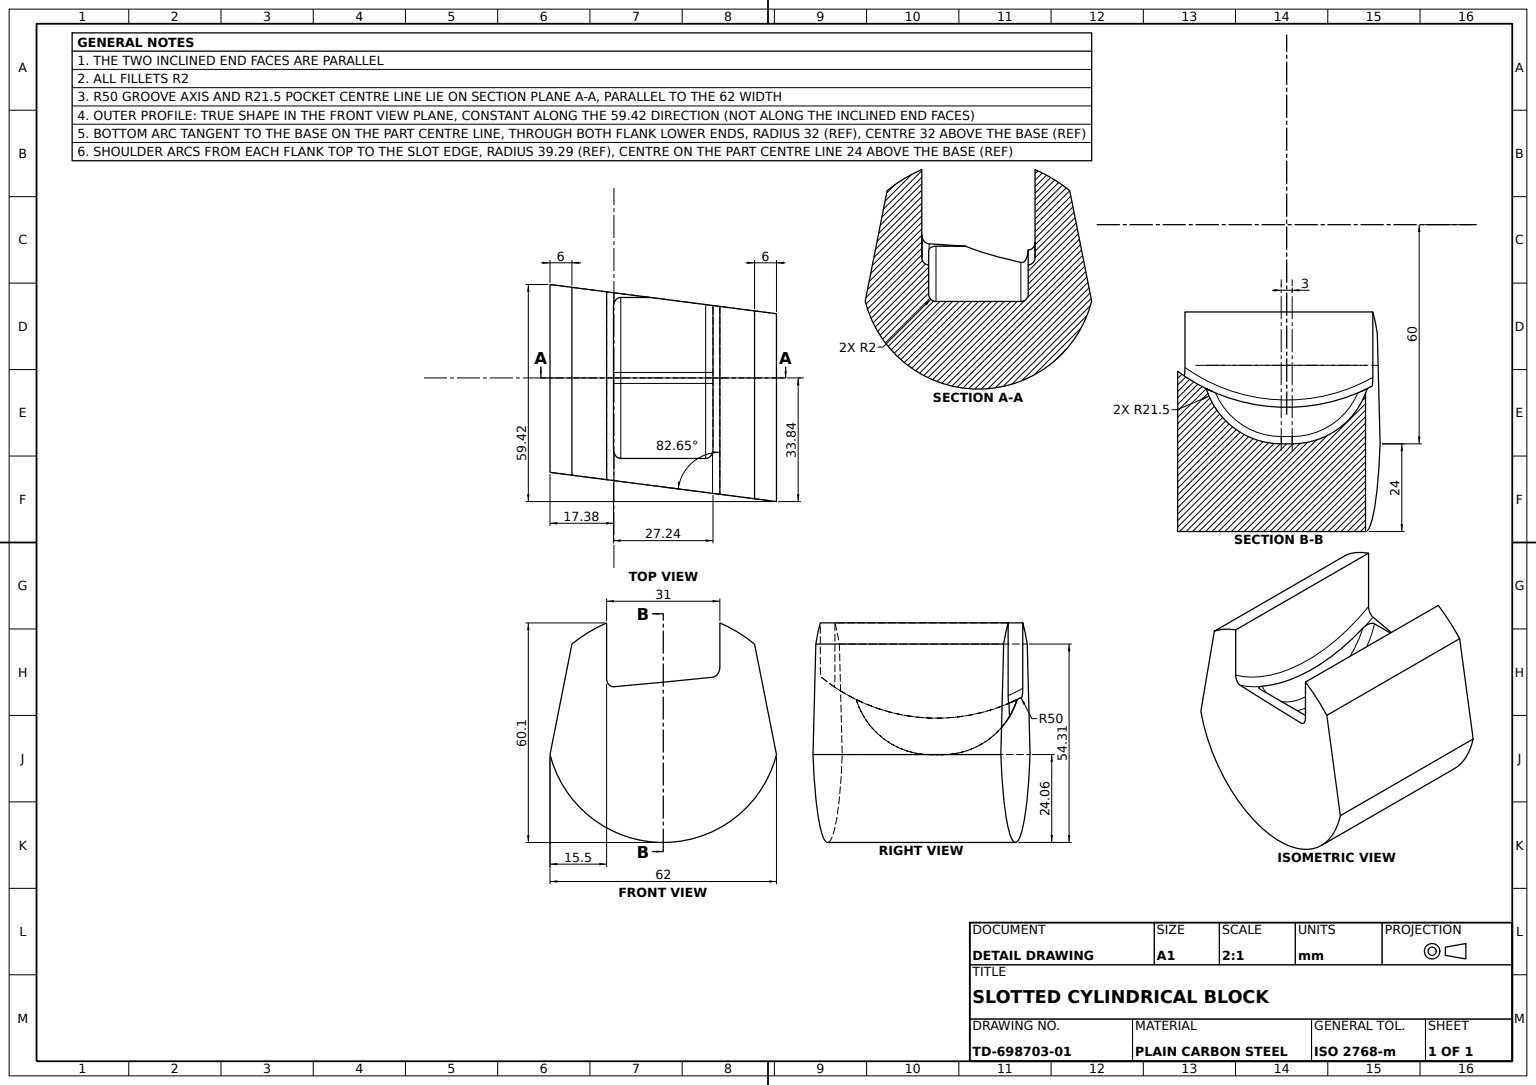
ISO-10303-21;
HEADER;
FILE_DESCRIPTION((''),'2;1');
FILE_NAME('','',(''),(''),'','','');
FILE_SCHEMA(('AUTOMOTIVE_DESIGN'));
ENDSEC;
DATA;
#1=APPLICATION_CONTEXT('');
#2=PRODUCT_CONTEXT('',#1,'mechanical');
#3=PRODUCT('','','',(#2));
#4=PRODUCT_DEFINITION_FORMATION('','',#3);
#5=PRODUCT_DEFINITION_CONTEXT('',#1,'design');
#6=PRODUCT_DEFINITION('','',#4,#5);
#7=PRODUCT_DEFINITION_SHAPE('','',#6);
#8=(LENGTH_UNIT()NAMED_UNIT(*)SI_UNIT(.MILLI.,.METRE.));
#9=(NAMED_UNIT(*)PLANE_ANGLE_UNIT()SI_UNIT($,.RADIAN.));
#10=(NAMED_UNIT(*)SI_UNIT($,.STERADIAN.)SOLID_ANGLE_UNIT());
#11=UNCERTAINTY_MEASURE_WITH_UNIT(LENGTH_MEASURE(1.E-05),#8,'distance_accuracy_value','');
#12=(GEOMETRIC_REPRESENTATION_CONTEXT(3)GLOBAL_UNCERTAINTY_ASSIGNED_CONTEXT((#11))GLOBAL_UNIT_ASSIGNED_CONTEXT((#8,#9,#10))REPRESENTATION_CONTEXT('',''));
#13=CARTESIAN_POINT('',(-18.473954,14.336783,15.994802));
#14=VERTEX_POINT('',#13);
#15=CARTESIAN_POINT('',(-20.362396,15.114804,14.342817));
#16=VERTEX_POINT('',#15);
#17=CARTESIAN_POINT('',(-18.689041,14.430126,15.963075));
#18=CARTESIAN_POINT('',(-18.897886,14.521165,15.909071));
#19=CARTESIAN_POINT('',(-19.30142,14.696555,15.748583));
#20=CARTESIAN_POINT('',(-19.49775,14.781622,15.64043));
#21=CARTESIAN_POINT('',(-19.848556,14.930594,15.366461));
#22=CARTESIAN_POINT('',(-20.007036,14.996145,15.196935));
#23=CARTESIAN_POINT('',(-20.188253,15.065265,14.902132));
#24=CARTESIAN_POINT('',(-20.2402,15.083776,14.795247));
#25=CARTESIAN_POINT('',(-20.319259,15.108385,14.575109));
#26=CARTESIAN_POINT('',(-20.347138,15.114804,14.461099));
#27=B_SPLINE_CURVE_WITH_KNOTS('',3,(#13,#17,#18,#19,#20,#21,#22,#23,#24,#25,#26,#15),.UNSPECIFIED.,.F.,.F.,(4,2,2,2,2,4),(0.,0.000701273,0.001402546,0.002103819,0.002454455,0.002805092),.UNSPECIFIED.);
#28=EDGE_CURVE('',#14,#16,#27,.T.);
#29=ORIENTED_EDGE('',*,*,#28,.F.);
#30=CARTESIAN_POINT('',(-17.578806,13.955249,16.000331));
#31=VERTEX_POINT('',#30);
#32=CARTESIAN_POINT('',(-17.877359,14.082612,16.038841));
#33=CARTESIAN_POINT('',(-18.176622,14.207749,16.038661));
#34=B_SPLINE_CURVE_WITH_KNOTS('',3,(#30,#32,#33,#13),.UNSPECIFIED.,.F.,.F.,(4,4),(0.,0.000973082),.UNSPECIFIED.);
#35=EDGE_CURVE('',#31,#14,#34,.T.);
#36=ORIENTED_EDGE('',*,*,#35,.F.);
#37=CARTESIAN_POINT('',(0.254734,2.,13.699982));
#38=VERTEX_POINT('',#37);
#39=CARTESIAN_POINT('',(0.254734,21.5,13.699982));
#40=DIRECTION('',(-0.127930151,0.,-0.99178318));
#41=DIRECTION('',(-0.99178318,0.,0.127930151));
#42=AXIS2_PLACEMENT_3D('',#39,#40,#41);
#43=CIRCLE('',#42,19.5);
#44=EDGE_CURVE('',#38,#31,#43,.T.);
#45=ORIENTED_EDGE('',*,*,#44,.F.);
#46=CARTESIAN_POINT('',(-0.001126,0.,11.716416));
#47=VERTEX_POINT('',#46);
#48=CARTESIAN_POINT('',(-0.001126,2.,11.716416));
#49=DIRECTION('',(0.99178318,0.,-0.127930151));
#50=AXIS2_PLACEMENT_3D('',#48,#49,#40);
#51=CIRCLE('',#50,2.);
#52=EDGE_CURVE('',#38,#47,#51,.T.);
#53=ORIENTED_EDGE('',*,*,#52,.T.);
#54=CARTESIAN_POINT('',(-0.001126,21.5,11.716416));
#55=DIRECTION('',(0.127930151,0.,0.99178318));
#56=AXIS2_PLACEMENT_3D('',#54,#55,#41);
#57=CIRCLE('',#56,21.5);
#58=EDGE_CURVE('',#16,#47,#57,.T.);
#59=ORIENTED_EDGE('',*,*,#58,.F.);
#60=EDGE_LOOP('',(#29,#36,#45,#53,#59));
#61=FACE_OUTER_BOUND('',#60,.T.);
#62=AXIS2_PLACEMENT_3D('',#54,#40,#41);
#63=TOROIDAL_SURFACE('',#62,19.5,2.);
#64=ADVANCED_FACE('',(#61),#63,.F.);
#65=CARTESIAN_POINT('',(29.6,20.902602,11.810311));
#66=VERTEX_POINT('',#65);
#67=CARTESIAN_POINT('',(-21.4,18.189213,18.388803));
#68=VERTEX_POINT('',#67);
#69=CARTESIAN_POINT('',(1.982917,60.,15.372639));
#70=AXIS2_PLACEMENT_3D('',#69,#40,#41);
#71=CIRCLE('',#70,48.);
#72=EDGE_CURVE('',#66,#68,#71,.T.);
#73=ORIENTED_EDGE('',*,*,#72,.T.);
#74=CARTESIAN_POINT('',(-21.4,36.103381,18.388803));
#75=VERTEX_POINT('',#74);
#76=CARTESIAN_POINT('',(-21.4,-24.,18.388803));
#77=DIRECTION('',(0.,-1.,0.));
#78=VECTOR('',#77,1000.);
#79=LINE('',#76,#78);
#80=EDGE_CURVE('',#75,#68,#79,.T.);
#81=ORIENTED_EDGE('',*,*,#80,.F.);
#82=CARTESIAN_POINT('',(29.6,36.103381,11.810311));
#83=VERTEX_POINT('',#82);
#84=CARTESIAN_POINT('',(138.187319,36.103381,-2.196372));
#85=VECTOR('',#49,1000.);
#86=LINE('',#84,#85);
#87=EDGE_CURVE('',#75,#83,#86,.T.);
#88=ORIENTED_EDGE('',*,*,#87,.T.);
#89=CARTESIAN_POINT('',(29.6,0.,11.810311));
#90=DIRECTION('',(0.,1.,0.));
#91=VECTOR('',#90,1000.);
#92=LINE('',#89,#91);
#93=EDGE_CURVE('',#66,#83,#92,.T.);
#94=ORIENTED_EDGE('',*,*,#93,.F.);
#95=EDGE_LOOP('',(#73,#81,#88,#94));
#96=FACE_OUTER_BOUND('',#95,.T.);
#97=PLANE('',#70);
#98=ADVANCED_FACE('',(#96),#97,.T.);
#99=CARTESIAN_POINT('',(-21.4,36.103381,-12.868029));
#100=VERTEX_POINT('',#99);
#101=CARTESIAN_POINT('',(-21.4,16.174165,-12.868029));
#102=VERTEX_POINT('',#101);
#103=CARTESIAN_POINT('',(-21.4,-24.,-12.868029));
#104=LINE('',#103,#78);
#105=EDGE_CURVE('',#100,#102,#104,.T.);
#106=ORIENTED_EDGE('',*,*,#105,.T.);
#107=CARTESIAN_POINT('',(29.6,24.084504,-19.446521));
#108=VERTEX_POINT('',#107);
#109=CARTESIAN_POINT('',(-1.982917,60.,-15.372639));
#110=AXIS2_PLACEMENT_3D('',#109,#55,#41);
#111=CIRCLE('',#110,48.);
#112=EDGE_CURVE('',#102,#108,#111,.T.);
#113=ORIENTED_EDGE('',*,*,#112,.T.);
#114=CARTESIAN_POINT('',(29.6,36.103381,-19.446521));
#115=VERTEX_POINT('',#114);
#116=CARTESIAN_POINT('',(29.6,0.,-19.446521));
#117=LINE('',#116,#91);
#118=EDGE_CURVE('',#108,#115,#117,.T.);
#119=ORIENTED_EDGE('',*,*,#118,.T.);
#120=CARTESIAN_POINT('',(134.221484,36.103381,-32.94165));
#121=LINE('',#120,#85);
#122=EDGE_CURVE('',#100,#115,#121,.T.);
#123=ORIENTED_EDGE('',*,*,#122,.F.);
#124=EDGE_LOOP('',(#106,#113,#119,#123));
#125=FACE_OUTER_BOUND('',#124,.T.);
#126=AXIS2_PLACEMENT_3D('',#109,#40,#41);
#127=PLANE('',#126);
#128=ADVANCED_FACE('',(#125),#127,.F.);
#129=ORIENTED_EDGE('',*,*,#44,.T.);
#130=CARTESIAN_POINT('',(21.063623,13.955249,11.015843));
#131=VERTEX_POINT('',#130);
#132=CARTESIAN_POINT('',(1.742409,60.,13.508087));
#133=AXIS2_PLACEMENT_3D('',#132,#55,#41);
#134=CIRCLE('',#133,49.996397);
#135=EDGE_CURVE('',#31,#131,#134,.T.);
#136=ORIENTED_EDGE('',*,*,#135,.T.);
#137=CARTESIAN_POINT('',(3.230083,2.,13.316192));
#138=VERTEX_POINT('',#137);
#139=CARTESIAN_POINT('',(3.230083,21.5,13.316192));
#140=AXIS2_PLACEMENT_3D('',#139,#40,#41);
#141=CIRCLE('',#140,19.5);
#142=EDGE_CURVE('',#131,#138,#141,.T.);
#143=ORIENTED_EDGE('',*,*,#142,.T.);
#144=VECTOR('',#41,1000.);
#145=LINE('',#137,#144);
#146=EDGE_CURVE('',#138,#38,#145,.T.);
#147=ORIENTED_EDGE('',*,*,#146,.T.);
#148=EDGE_LOOP('',(#129,#136,#143,#147));
#149=FACE_OUTER_BOUND('',#148,.T.);
#150=PLANE('',#140);
#151=ADVANCED_FACE('',(#149),#150,.T.);
#152=CARTESIAN_POINT('',(-21.063623,13.955249,-11.015843));
#153=VERTEX_POINT('',#152);
#154=CARTESIAN_POINT('',(17.578806,13.955249,-16.000331));
#155=VERTEX_POINT('',#154);
#156=CARTESIAN_POINT('',(-1.742409,60.,-13.508087));
#157=AXIS2_PLACEMENT_3D('',#156,#55,#41);
#158=CIRCLE('',#157,49.996397);
#159=EDGE_CURVE('',#153,#155,#158,.T.);
#160=ORIENTED_EDGE('',*,*,#159,.F.);
#161=CARTESIAN_POINT('',(-3.230083,2.,-13.316192));
#162=VERTEX_POINT('',#161);
#163=CARTESIAN_POINT('',(-3.230083,21.5,-13.316192));
#164=AXIS2_PLACEMENT_3D('',#163,#55,#41);
#165=CIRCLE('',#164,19.5);
#166=EDGE_CURVE('',#153,#162,#165,.T.);
#167=ORIENTED_EDGE('',*,*,#166,.T.);
#168=CARTESIAN_POINT('',(-0.254734,2.,-13.699982));
#169=VERTEX_POINT('',#168);
#170=LINE('',#168,#85);
#171=EDGE_CURVE('',#162,#169,#170,.T.);
#172=ORIENTED_EDGE('',*,*,#171,.T.);
#173=CARTESIAN_POINT('',(-0.254734,21.5,-13.699982));
#174=AXIS2_PLACEMENT_3D('',#173,#55,#41);
#175=CIRCLE('',#174,19.5);
#176=EDGE_CURVE('',#169,#155,#175,.T.);
#177=ORIENTED_EDGE('',*,*,#176,.T.);
#178=EDGE_LOOP('',(#160,#167,#172,#177));
#179=FACE_OUTER_BOUND('',#178,.T.);
#180=AXIS2_PLACEMENT_3D('',#173,#40,#41);
#181=PLANE('',#180);
#182=ADVANCED_FACE('',(#179),#181,.F.);
#183=CARTESIAN_POINT('',(29.6,30.310132,-29.025228));
#184=VERTEX_POINT('',#183);
#185=CARTESIAN_POINT('',(29.6,32.686123,-26.120697));
#186=CARTESIAN_POINT('',(29.6,34.630266,-22.906201));
#187=(BOUNDED_CURVE()B_SPLINE_CURVE(3,(#183,#185,#186,#114),.UNSPECIFIED.,.F.,.T.)B_SPLINE_CURVE_WITH_KNOTS((4,4),(4.022703962,4.306862693),.UNSPECIFIED.)CURVE()GEOMETRIC_REPRESENTATION_ITEM()RATIONAL_B_SPLINE_CURVE((1.,0.993282463,0.993282463,1.))REPRESENTATION_ITEM(''));
#188=EDGE_CURVE('',#184,#115,#187,.T.);
#189=ORIENTED_EDGE('',*,*,#188,.T.);
#190=ORIENTED_EDGE('',*,*,#118,.F.);
#191=CARTESIAN_POINT('',(29.6,21.240655,-17.429951));
#192=VERTEX_POINT('',#191);
#193=CARTESIAN_POINT('',(29.6,23.766192,-19.446521));
#194=CARTESIAN_POINT('',(29.6,23.453843,-19.404951));
#195=CARTESIAN_POINT('',(29.6,22.841292,-19.237101));
#196=CARTESIAN_POINT('',(29.6,22.551273,-19.113224));
#197=CARTESIAN_POINT('',(29.6,22.152824,-18.861976));
#198=CARTESIAN_POINT('',(29.6,22.02448,-18.765714));
#199=CARTESIAN_POINT('',(29.6,21.78991,-18.552291));
#200=CARTESIAN_POINT('',(29.6,21.683573,-18.435599));
#201=CARTESIAN_POINT('',(29.6,21.403413,-18.050105));
#202=CARTESIAN_POINT('',(29.6,21.273916,-17.748985));
#203=B_SPLINE_CURVE_WITH_KNOTS('',3,(#107,#193,#194,#195,#196,#197,#198,#199,#200,#201,#202,#191),.UNSPECIFIED.,.F.,.F.,(4,2,2,2,2,4),(0.,0.000945263,0.001890527,0.002363159,0.00283579,0.003781054),.UNSPECIFIED.);
#204=EDGE_CURVE('',#108,#192,#203,.T.);
#205=ORIENTED_EDGE('',*,*,#204,.T.);
#206=CARTESIAN_POINT('',(29.6,18.645766,9.793741));
#207=VERTEX_POINT('',#206);
#208=CARTESIAN_POINT('',(29.6,19.460005,0.428199));
#209=CARTESIAN_POINT('',(29.6,20.325513,-8.652077));
#210=(BOUNDED_CURVE()B_SPLINE_CURVE(3,(#206,#208,#209,#191),.UNSPECIFIED.,.F.,.T.)B_SPLINE_CURVE_WITH_KNOTS((4,4),(5.309284293,5.396174423),.UNSPECIFIED.)CURVE()GEOMETRIC_REPRESENTATION_ITEM()RATIONAL_B_SPLINE_CURVE((1.,0.999370941,0.999370941,1.))REPRESENTATION_ITEM(''));
#211=EDGE_CURVE('',#207,#192,#210,.T.);
#212=ORIENTED_EDGE('',*,*,#211,.F.);
#213=CARTESIAN_POINT('',(29.6,18.633344,9.936629));
#214=CARTESIAN_POINT('',(29.6,18.639072,10.07802));
#215=CARTESIAN_POINT('',(29.6,18.686934,10.357802));
#216=CARTESIAN_POINT('',(29.6,18.729721,10.49589));
#217=CARTESIAN_POINT('',(29.6,18.846936,10.753352));
#218=CARTESIAN_POINT('',(29.6,18.922887,10.876228));
#219=CARTESIAN_POINT('',(29.6,19.099554,11.098621));
#220=CARTESIAN_POINT('',(29.6,19.200183,11.198892));
#221=CARTESIAN_POINT('',(29.6,19.423027,11.378495));
#222=CARTESIAN_POINT('',(29.6,19.54213,11.455395));
#223=CARTESIAN_POINT('',(29.6,19.793637,11.586856));
#224=CARTESIAN_POINT('',(29.6,19.926801,11.641427));
#225=CARTESIAN_POINT('',(29.6,20.332291,11.769488));
#226=CARTESIAN_POINT('',(29.6,20.61683,11.810311));
#227=B_SPLINE_CURVE_WITH_KNOTS('',3,(#206,#213,#214,#215,#216,#217,#218,#219,#220,#221,#222,#223,#224,#225,#226,#65),.UNSPECIFIED.,.F.,.F.,(4,2,2,2,2,2,2,4),(0.,0.000424152,0.000848305,0.001272457,0.001696609,0.002120761,0.002544914,0.003393218),.UNSPECIFIED.);
#228=EDGE_CURVE('',#207,#66,#227,.T.);
#229=ORIENTED_EDGE('',*,*,#228,.T.);
#230=ORIENTED_EDGE('',*,*,#93,.T.);
#231=CARTESIAN_POINT('',(29.6,30.310132,21.389017));
#232=VERTEX_POINT('',#231);
#233=CARTESIAN_POINT('',(29.6,34.630266,15.269991));
#234=CARTESIAN_POINT('',(29.6,32.686123,18.484487));
#235=(BOUNDED_CURVE()B_SPLINE_CURVE(3,(#82,#233,#234,#231),.UNSPECIFIED.,.F.,.F.)B_SPLINE_CURVE_WITH_KNOTS((4,4),(5.117915268,5.402073999),.UNSPECIFIED.)CURVE()GEOMETRIC_REPRESENTATION_ITEM()RATIONAL_B_SPLINE_CURVE((1.,0.993282463,0.993282463,1.))REPRESENTATION_ITEM(''));
#236=EDGE_CURVE('',#83,#232,#235,.T.);
#237=ORIENTED_EDGE('',*,*,#236,.T.);
#238=CARTESIAN_POINT('',(29.6,0.062746,27.438727));
#239=VERTEX_POINT('',#238);
#240=CARTESIAN_POINT('',(29.6,-357239.520955,71478.097788));
#241=DIRECTION('',(0.,0.980579228,-0.196123373));
#242=VECTOR('',#241,1000.);
#243=LINE('',#240,#242);
#244=EDGE_CURVE('',#239,#232,#243,.T.);
#245=ORIENTED_EDGE('',*,*,#244,.F.);
#246=CARTESIAN_POINT('',(29.6,0.062746,-35.074937));
#247=VERTEX_POINT('',#246);
#248=CARTESIAN_POINT('',(29.6,-40.083881,17.074404));
#249=CARTESIAN_POINT('',(29.6,-40.083881,-24.710615));
#250=(BOUNDED_CURVE()B_SPLINE_CURVE(3,(#238,#248,#249,#246),.UNSPECIFIED.,.F.,.T.)B_SPLINE_CURVE_WITH_KNOTS((4,4),(0.250655662,2.890936991),.UNSPECIFIED.)CURVE()GEOMETRIC_REPRESENTATION_ITEM()RATIONAL_B_SPLINE_CURVE((1.,0.49869279,0.49869279,1.))REPRESENTATION_ITEM(''));
#251=EDGE_CURVE('',#239,#247,#250,.T.);
#252=ORIENTED_EDGE('',*,*,#251,.T.);
#253=CARTESIAN_POINT('',(29.6,-203394.108466,-40715.470519));
#254=DIRECTION('',(0.,-0.980579228,-0.196123373));
#255=VECTOR('',#254,1000.);
#256=LINE('',#253,#255);
#257=EDGE_CURVE('',#184,#247,#256,.T.);
#258=ORIENTED_EDGE('',*,*,#257,.F.);
#259=EDGE_LOOP('',(#189,#190,#205,#212,#229,#230,#237,#245,#252,#258));
#260=FACE_OUTER_BOUND('',#259,.T.);
#261=CARTESIAN_POINT('',(29.6,0.,0.));
#262=DIRECTION('',(1.,0.,0.));
#263=DIRECTION('',(0.,0.,-1.));
#264=AXIS2_PLACEMENT_3D('',#261,#262,#263);
#265=PLANE('',#264);
#266=ADVANCED_FACE('',(#260),#265,.T.);
#267=CARTESIAN_POINT('',(-21.4,30.310132,-22.446736));
#268=VERTEX_POINT('',#267);
#269=CARTESIAN_POINT('',(133.006148,30.310132,-42.363591));
#270=LINE('',#269,#144);
#271=EDGE_CURVE('',#184,#268,#270,.T.);
#272=ORIENTED_EDGE('',*,*,#271,.T.);
#273=CARTESIAN_POINT('',(-21.4,32.654041,-19.581424));
#274=CARTESIAN_POINT('',(-21.4,34.610635,-16.373814));
#275=(BOUNDED_CURVE()B_SPLINE_CURVE(3,(#267,#273,#274,#99),.UNSPECIFIED.,.F.,.T.)B_SPLINE_CURVE_WITH_KNOTS((4,4),(0.,0.213820488),.UNSPECIFIED.)CURVE()GEOMETRIC_REPRESENTATION_ITEM()RATIONAL_B_SPLINE_CURVE((1.,0.967420382,0.941806955,0.923159716))REPRESENTATION_ITEM(''));
#276=EDGE_CURVE('',#268,#100,#275,.T.);
#277=ORIENTED_EDGE('',*,*,#276,.T.);
#278=ORIENTED_EDGE('',*,*,#122,.T.);
#279=ORIENTED_EDGE('',*,*,#188,.F.);
#280=EDGE_LOOP('',(#272,#277,#278,#279));
#281=FACE_OUTER_BOUND('',#280,.T.);
#282=CARTESIAN_POINT('',(136.204402,0.,-17.569011));
#283=AXIS2_PLACEMENT_3D('',#282,#41,#55);
#284=CYLINDRICAL_SURFACE('',#283,39.29);
#285=ADVANCED_FACE('',(#281),#284,.T.);
#286=ORIENTED_EDGE('',*,*,#28,.T.);
#287=CARTESIAN_POINT('',(-21.4,15.114804,6.298751));
#288=VERTEX_POINT('',#287);
#289=CARTESIAN_POINT('',(-21.848944,15.114804,2.818296));
#290=VECTOR('',#40,1000.);
#291=LINE('',#289,#290);
#292=EDGE_CURVE('',#16,#288,#291,.T.);
#293=ORIENTED_EDGE('',*,*,#292,.T.);
#294=CARTESIAN_POINT('',(-21.4,15.770598,16.372233));
#295=VERTEX_POINT('',#294);
#296=CARTESIAN_POINT('',(-21.4,15.327182,9.681171));
#297=CARTESIAN_POINT('',(-21.4,15.545796,13.039232));
#298=(BOUNDED_CURVE()B_SPLINE_CURVE(3,(#287,#296,#297,#294),.UNSPECIFIED.,.F.,.T.)B_SPLINE_CURVE_WITH_KNOTS((4,4),(2.027062377,2.055982717),.UNSPECIFIED.)CURVE()GEOMETRIC_REPRESENTATION_ITEM()RATIONAL_B_SPLINE_CURVE((1.,0.999930302,0.999930302,1.))REPRESENTATION_ITEM(''));
#299=EDGE_CURVE('',#288,#295,#298,.T.);
#300=ORIENTED_EDGE('',*,*,#299,.T.);
#301=CARTESIAN_POINT('',(1.727057,60.,13.389073));
#302=AXIS2_PLACEMENT_3D('',#301,#55,#41);
#303=CIRCLE('',#302,50.);
#304=EDGE_CURVE('',#295,#14,#303,.T.);
#305=ORIENTED_EDGE('',*,*,#304,.T.);
#306=EDGE_LOOP('',(#286,#293,#300,#305));
#307=FACE_OUTER_BOUND('',#306,.T.);
#308=CYLINDRICAL_SURFACE('',#70,50.);
#309=ADVANCED_FACE('',(#307),#308,.F.);
#310=ORIENTED_EDGE('',*,*,#251,.F.);
#311=CARTESIAN_POINT('',(-21.4,0.062746,34.017219));
#312=VERTEX_POINT('',#311);
#313=CARTESIAN_POINT('',(133.006148,0.062746,14.100364));
#314=LINE('',#313,#144);
#315=EDGE_CURVE('',#239,#312,#314,.T.);
#316=ORIENTED_EDGE('',*,*,#315,.T.);
#317=CARTESIAN_POINT('',(-21.4,0.062746,-28.496445));
#318=VERTEX_POINT('',#317);
#319=CARTESIAN_POINT('',(-21.4,-40.083881,23.652896));
#320=CARTESIAN_POINT('',(-21.4,-40.083881,-18.132123));
#321=(BOUNDED_CURVE()B_SPLINE_CURVE(3,(#311,#319,#320,#317),.UNSPECIFIED.,.F.,.T.)B_SPLINE_CURVE_WITH_KNOTS((4,4),(0.,1.),.UNSPECIFIED.)CURVE()GEOMETRIC_REPRESENTATION_ITEM()RATIONAL_B_SPLINE_CURVE((1.,0.49869279,0.49869279,1.))REPRESENTATION_ITEM(''));
#322=EDGE_CURVE('',#312,#318,#321,.T.);
#323=ORIENTED_EDGE('',*,*,#322,.T.);
#324=CARTESIAN_POINT('',(133.006148,0.062746,-48.4133));
#325=LINE('',#324,#144);
#326=EDGE_CURVE('',#247,#318,#325,.T.);
#327=ORIENTED_EDGE('',*,*,#326,.F.);
#328=EDGE_LOOP('',(#310,#316,#323,#327));
#329=FACE_OUTER_BOUND('',#328,.T.);
#330=CARTESIAN_POINT('',(129.040313,8.,-16.644915));
#331=AXIS2_PLACEMENT_3D('',#330,#41,#55);
#332=CYLINDRICAL_SURFACE('',#331,32.);
#333=ADVANCED_FACE('',(#329),#332,.T.);
#334=ORIENTED_EDGE('',*,*,#304,.F.);
#335=CARTESIAN_POINT('',(-21.4,17.898171,18.388803));
#336=CARTESIAN_POINT('',(-21.4,17.616355,18.341888));
#337=CARTESIAN_POINT('',(-21.4,17.206976,18.203635));
#338=CARTESIAN_POINT('',(-21.4,17.072518,18.145473));
#339=CARTESIAN_POINT('',(-21.4,16.819473,18.009465));
#340=CARTESIAN_POINT('',(-21.4,16.699428,17.931246));
#341=CARTESIAN_POINT('',(-21.4,16.473123,17.753072));
#342=CARTESIAN_POINT('',(-21.4,16.366372,17.652165));
#343=CARTESIAN_POINT('',(-21.4,16.177579,17.43572));
#344=CARTESIAN_POINT('',(-21.4,16.094216,17.319396));
#345=CARTESIAN_POINT('',(-21.4,15.951586,17.069055));
#346=CARTESIAN_POINT('',(-21.4,15.89248,16.934121));
#347=CARTESIAN_POINT('',(-21.4,15.80749,16.659421));
#348=CARTESIAN_POINT('',(-21.4,15.780434,16.518063));
#349=B_SPLINE_CURVE_WITH_KNOTS('',3,(#67,#335,#336,#337,#338,#339,#340,#341,#342,#343,#344,#345,#346,#347,#348,#294),.UNSPECIFIED.,.F.,.F.,(4,2,2,2,2,2,2,4),(0.,0.00085672,0.00128508,0.00171344,0.002141801,0.002570161,0.002998521,0.003426881),.UNSPECIFIED.);
#350=EDGE_CURVE('',#68,#295,#349,.T.);
#351=ORIENTED_EDGE('',*,*,#350,.F.);
#352=ORIENTED_EDGE('',*,*,#72,.F.);
#353=ORIENTED_EDGE('',*,*,#228,.F.);
#354=CARTESIAN_POINT('',(21.928068,14.336783,10.783344));
#355=VERTEX_POINT('',#354);
#356=EDGE_CURVE('',#355,#207,#303,.T.);
#357=ORIENTED_EDGE('',*,*,#356,.F.);
#358=CARTESIAN_POINT('',(21.651598,14.207749,10.901217));
#359=CARTESIAN_POINT('',(21.362176,14.082612,10.977332));
#360=B_SPLINE_CURVE_WITH_KNOTS('',3,(#354,#358,#359,#130),.UNSPECIFIED.,.F.,.F.,(4,4),(0.,0.000973082),.UNSPECIFIED.);
#361=EDGE_CURVE('',#355,#131,#360,.T.);
#362=ORIENTED_EDGE('',*,*,#361,.T.);
#363=ORIENTED_EDGE('',*,*,#135,.F.);
#364=ORIENTED_EDGE('',*,*,#35,.T.);
#365=EDGE_LOOP('',(#334,#351,#352,#353,#357,#362,#363,#364));
#366=FACE_OUTER_BOUND('',#365,.T.);
#367=AXIS2_PLACEMENT_3D('',#301,#40,#41);
#368=TOROIDAL_SURFACE('',#367,48.,2.);
#369=ADVANCED_FACE('',(#366),#368,.F.);
#370=CARTESIAN_POINT('',(2.974223,0.,11.332625));
#371=VERTEX_POINT('',#370);
#372=CARTESIAN_POINT('',(23.335492,15.114804,8.706224));
#373=VERTEX_POINT('',#372);
#374=CARTESIAN_POINT('',(2.974223,21.5,11.332625));
#375=AXIS2_PLACEMENT_3D('',#374,#55,#41);
#376=CIRCLE('',#375,21.5);
#377=EDGE_CURVE('',#371,#373,#376,.T.);
#378=ORIENTED_EDGE('',*,*,#377,.T.);
#379=CARTESIAN_POINT('',(20.362396,15.114804,-14.342817));
#380=VERTEX_POINT('',#379);
#381=CARTESIAN_POINT('',(21.848944,15.114804,-2.818296));
#382=VECTOR('',#55,1000.);
#383=LINE('',#381,#382);
#384=EDGE_CURVE('',#380,#373,#383,.T.);
#385=ORIENTED_EDGE('',*,*,#384,.F.);
#386=CARTESIAN_POINT('',(0.001126,0.,-11.716416));
#387=VERTEX_POINT('',#386);
#388=CARTESIAN_POINT('',(0.001126,21.5,-11.716416));
#389=AXIS2_PLACEMENT_3D('',#388,#40,#41);
#390=CIRCLE('',#389,21.5);
#391=EDGE_CURVE('',#380,#387,#390,.T.);
#392=ORIENTED_EDGE('',*,*,#391,.T.);
#393=CARTESIAN_POINT('',(3.230083,0.,13.316192));
#394=LINE('',#393,#290);
#395=EDGE_CURVE('',#371,#387,#394,.T.);
#396=ORIENTED_EDGE('',*,*,#395,.F.);
#397=EDGE_LOOP('',(#378,#385,#392,#396));
#398=FACE_OUTER_BOUND('',#397,.T.);
#399=CYLINDRICAL_SURFACE('',#140,21.5);
#400=ADVANCED_FACE('',(#398),#399,.F.);
#401=ORIENTED_EDGE('',*,*,#257,.T.);
#402=ORIENTED_EDGE('',*,*,#326,.T.);
#403=CARTESIAN_POINT('',(-21.4,-203391.543306,-40708.378975));
#404=LINE('',#403,#255);
#405=EDGE_CURVE('',#268,#318,#404,.T.);
#406=ORIENTED_EDGE('',*,*,#405,.F.);
#407=ORIENTED_EDGE('',*,*,#271,.F.);
#408=EDGE_LOOP('',(#401,#402,#406,#407));
#409=FACE_OUTER_BOUND('',#408,.T.);
#410=CARTESIAN_POINT('',(133.006148,-203391.543306,-40728.29583));
#411=DIRECTION('',(-0.125485152,0.194573115,-0.972828237));
#412=DIRECTION('',(0.,0.980579228,0.196123373));
#413=AXIS2_PLACEMENT_3D('',#410,#411,#412);
#414=PLANE('',#413);
#415=ADVANCED_FACE('',(#409),#414,.T.);
#416=CARTESIAN_POINT('',(18.473954,14.336783,-15.994802));
#417=VERTEX_POINT('',#416);
#418=CARTESIAN_POINT('',(18.689041,14.430126,-15.963075));
#419=CARTESIAN_POINT('',(18.897886,14.521165,-15.909071));
#420=CARTESIAN_POINT('',(19.30142,14.696555,-15.748583));
#421=CARTESIAN_POINT('',(19.49775,14.781622,-15.64043));
#422=CARTESIAN_POINT('',(19.848556,14.930594,-15.366461));
#423=CARTESIAN_POINT('',(20.007036,14.996145,-15.196935));
#424=CARTESIAN_POINT('',(20.188253,15.065265,-14.902132));
#425=CARTESIAN_POINT('',(20.2402,15.083776,-14.795247));
#426=CARTESIAN_POINT('',(20.319259,15.108385,-14.575109));
#427=CARTESIAN_POINT('',(20.347138,15.114804,-14.461099));
#428=B_SPLINE_CURVE_WITH_KNOTS('',3,(#416,#418,#419,#420,#421,#422,#423,#424,#425,#426,#427,#379),.UNSPECIFIED.,.F.,.F.,(4,2,2,2,2,4),(0.,0.000701273,0.001402546,0.002103819,0.002454455,0.002805092),.UNSPECIFIED.);
#429=EDGE_CURVE('',#417,#380,#428,.T.);
#430=ORIENTED_EDGE('',*,*,#429,.F.);
#431=CARTESIAN_POINT('',(17.877359,14.082612,-16.038841));
#432=CARTESIAN_POINT('',(18.176622,14.207749,-16.038661));
#433=B_SPLINE_CURVE_WITH_KNOTS('',3,(#154,#431,#432,#416),.UNSPECIFIED.,.F.,.F.,(4,4),(0.,0.000973082),.UNSPECIFIED.);
#434=EDGE_CURVE('',#155,#417,#433,.T.);
#435=ORIENTED_EDGE('',*,*,#434,.F.);
#436=ORIENTED_EDGE('',*,*,#176,.F.);
#437=CARTESIAN_POINT('',(0.001126,2.,-11.716416));
#438=AXIS2_PLACEMENT_3D('',#437,#49,#40);
#439=CIRCLE('',#438,2.);
#440=EDGE_CURVE('',#387,#169,#439,.T.);
#441=ORIENTED_EDGE('',*,*,#440,.F.);
#442=ORIENTED_EDGE('',*,*,#391,.F.);
#443=EDGE_LOOP('',(#430,#435,#436,#441,#442));
#444=FACE_OUTER_BOUND('',#443,.T.);
#445=TOROIDAL_SURFACE('',#389,19.5,2.);
#446=ADVANCED_FACE('',(#444),#445,.F.);
#447=ORIENTED_EDGE('',*,*,#361,.F.);
#448=CARTESIAN_POINT('',(23.35075,15.114804,8.824508));
#449=CARTESIAN_POINT('',(23.352704,15.108385,8.941778));
#450=CARTESIAN_POINT('',(23.332157,15.083826,9.174458));
#451=CARTESIAN_POINT('',(23.309094,15.065347,9.290992));
#452=CARTESIAN_POINT('',(23.208491,14.996129,9.622715));
#453=CARTESIAN_POINT('',(23.098074,14.930508,9.826956));
#454=CARTESIAN_POINT('',(22.828597,14.781715,10.180555));
#455=CARTESIAN_POINT('',(22.666242,14.696694,10.334985));
#456=CARTESIAN_POINT('',(22.316437,14.521197,10.592814));
#457=CARTESIAN_POINT('',(22.12807,14.430129,10.698073));
#458=B_SPLINE_CURVE_WITH_KNOTS('',3,(#372,#448,#449,#450,#451,#452,#453,#454,#455,#456,#457,#354),.UNSPECIFIED.,.F.,.F.,(4,2,2,2,2,4),(0.,0.000351756,0.000703512,0.001407024,0.002110536,0.002814048),.UNSPECIFIED.);
#459=EDGE_CURVE('',#373,#355,#458,.T.);
#460=ORIENTED_EDGE('',*,*,#459,.F.);
#461=ORIENTED_EDGE('',*,*,#377,.F.);
#462=CARTESIAN_POINT('',(2.974223,2.,11.332625));
#463=AXIS2_PLACEMENT_3D('',#462,#49,#40);
#464=CIRCLE('',#463,2.);
#465=EDGE_CURVE('',#138,#371,#464,.T.);
#466=ORIENTED_EDGE('',*,*,#465,.F.);
#467=ORIENTED_EDGE('',*,*,#142,.F.);
#468=EDGE_LOOP('',(#447,#460,#461,#466,#467));
#469=FACE_OUTER_BOUND('',#468,.T.);
#470=AXIS2_PLACEMENT_3D('',#374,#40,#41);
#471=TOROIDAL_SURFACE('',#470,19.5,2.);
#472=ADVANCED_FACE('',(#469),#471,.F.);
#473=CARTESIAN_POINT('',(-2.974223,0.,-11.332625));
#474=VERTEX_POINT('',#473);
#475=CARTESIAN_POINT('',(0.254734,0.,13.699982));
#476=LINE('',#475,#290);
#477=EDGE_CURVE('',#47,#474,#476,.T.);
#478=ORIENTED_EDGE('',*,*,#477,.T.);
#479=CARTESIAN_POINT('',(-21.4,10.679101,-8.955884));
#480=VERTEX_POINT('',#479);
#481=CARTESIAN_POINT('',(-2.974223,21.5,-11.332625));
#482=AXIS2_PLACEMENT_3D('',#481,#40,#41);
#483=CIRCLE('',#482,21.5);
#484=EDGE_CURVE('',#474,#480,#483,.T.);
#485=ORIENTED_EDGE('',*,*,#484,.T.);
#486=CARTESIAN_POINT('',(-21.4,12.080892,-2.573772));
#487=CARTESIAN_POINT('',(-21.4,13.565766,2.532794));
#488=(BOUNDED_CURVE()B_SPLINE_CURVE(3,(#479,#486,#487,#287),.UNSPECIFIED.,.F.,.T.)B_SPLINE_CURVE_WITH_KNOTS((4,4),(2.614181925,2.840058096),.UNSPECIFIED.)CURVE()GEOMETRIC_REPRESENTATION_ITEM()RATIONAL_B_SPLINE_CURVE((1.,0.995752847,0.995752847,1.))REPRESENTATION_ITEM(''));
#489=EDGE_CURVE('',#480,#288,#488,.T.);
#490=ORIENTED_EDGE('',*,*,#489,.T.);
#491=ORIENTED_EDGE('',*,*,#292,.F.);
#492=ORIENTED_EDGE('',*,*,#58,.T.);
#493=EDGE_LOOP('',(#478,#485,#490,#491,#492));
#494=FACE_OUTER_BOUND('',#493,.T.);
#495=CYLINDRICAL_SURFACE('',#42,21.5);
#496=ADVANCED_FACE('',(#494),#495,.F.);
#497=ORIENTED_EDGE('',*,*,#87,.F.);
#498=CARTESIAN_POINT('',(-21.4,30.310132,27.967509));
#499=VERTEX_POINT('',#498);
#500=CARTESIAN_POINT('',(-21.4,34.610635,21.894588));
#501=CARTESIAN_POINT('',(-21.4,32.654041,25.102197));
#502=(BOUNDED_CURVE()B_SPLINE_CURVE(3,(#74,#500,#501,#498),.UNSPECIFIED.,.F.,.T.)B_SPLINE_CURVE_WITH_KNOTS((4,4),(0.786179512,1.),.UNSPECIFIED.)CURVE()GEOMETRIC_REPRESENTATION_ITEM()RATIONAL_B_SPLINE_CURVE((0.923159716,0.941806955,0.967420382,1.))REPRESENTATION_ITEM(''));
#503=EDGE_CURVE('',#75,#499,#502,.T.);
#504=ORIENTED_EDGE('',*,*,#503,.T.);
#505=CARTESIAN_POINT('',(133.006148,30.310132,8.050654));
#506=LINE('',#505,#144);
#507=EDGE_CURVE('',#232,#499,#506,.T.);
#508=ORIENTED_EDGE('',*,*,#507,.F.);
#509=ORIENTED_EDGE('',*,*,#236,.F.);
#510=EDGE_LOOP('',(#497,#504,#508,#509));
#511=FACE_OUTER_BOUND('',#510,.T.);
#512=ADVANCED_FACE('',(#511),#284,.T.);
#513=LINE('',#370,#85);
#514=EDGE_CURVE('',#47,#371,#513,.T.);
#515=ORIENTED_EDGE('',*,*,#514,.T.);
#516=ORIENTED_EDGE('',*,*,#395,.T.);
#517=LINE('',#473,#144);
#518=EDGE_CURVE('',#387,#474,#517,.T.);
#519=ORIENTED_EDGE('',*,*,#518,.T.);
#520=ORIENTED_EDGE('',*,*,#477,.F.);
#521=EDGE_LOOP('',(#515,#516,#519,#520));
#522=FACE_OUTER_BOUND('',#521,.T.);
#523=AXIS2_PLACEMENT_3D('',#393,#77,#262);
#524=PLANE('',#523);
#525=ADVANCED_FACE('',(#522),#524,.F.);
#526=ORIENTED_EDGE('',*,*,#514,.F.);
#527=ORIENTED_EDGE('',*,*,#52,.F.);
#528=ORIENTED_EDGE('',*,*,#146,.F.);
#529=ORIENTED_EDGE('',*,*,#465,.T.);
#530=EDGE_LOOP('',(#526,#527,#528,#529));
#531=FACE_OUTER_BOUND('',#530,.T.);
#532=AXIS2_PLACEMENT_3D('',#462,#41,#55);
#533=CYLINDRICAL_SURFACE('',#532,2.);
#534=ADVANCED_FACE('',(#531),#533,.F.);
#535=ORIENTED_EDGE('',*,*,#211,.T.);
#536=CARTESIAN_POINT('',(-1.727057,60.,-13.389073));
#537=AXIS2_PLACEMENT_3D('',#536,#40,#41);
#538=CIRCLE('',#537,50.);
#539=EDGE_CURVE('',#192,#417,#538,.T.);
#540=ORIENTED_EDGE('',*,*,#539,.T.);
#541=ORIENTED_EDGE('',*,*,#429,.T.);
#542=ORIENTED_EDGE('',*,*,#384,.T.);
#543=ORIENTED_EDGE('',*,*,#459,.T.);
#544=ORIENTED_EDGE('',*,*,#356,.T.);
#545=EDGE_LOOP('',(#535,#540,#541,#542,#543,#544));
#546=FACE_OUTER_BOUND('',#545,.T.);
#547=ADVANCED_FACE('',(#546),#308,.F.);
#548=ORIENTED_EDGE('',*,*,#507,.T.);
#549=CARTESIAN_POINT('',(-21.4,-357242.086115,71485.189332));
#550=LINE('',#549,#242);
#551=EDGE_CURVE('',#312,#499,#550,.T.);
#552=ORIENTED_EDGE('',*,*,#551,.F.);
#553=ORIENTED_EDGE('',*,*,#315,.F.);
#554=ORIENTED_EDGE('',*,*,#244,.T.);
#555=EDGE_LOOP('',(#548,#552,#553,#554));
#556=FACE_OUTER_BOUND('',#555,.T.);
#557=CARTESIAN_POINT('',(133.006148,-357242.086115,71465.272477));
#558=DIRECTION('',(0.125485152,0.194573115,0.972828237));
#559=DIRECTION('',(0.,-0.980579228,0.196123373));
#560=AXIS2_PLACEMENT_3D('',#557,#558,#559);
#561=PLANE('',#560);
#562=ADVANCED_FACE('',(#556),#561,.T.);
#563=CARTESIAN_POINT('',(-21.4,14.100138,-10.955274));
#564=VERTEX_POINT('',#563);
#565=CARTESIAN_POINT('',(-21.4,14.100196,-11.086339));
#566=CARTESIAN_POINT('',(-21.4,14.113986,-11.215856));
#567=CARTESIAN_POINT('',(-21.4,14.169453,-11.471745));
#568=CARTESIAN_POINT('',(-21.4,14.211517,-11.597831));
#569=CARTESIAN_POINT('',(-21.4,14.374133,-11.953209));
#570=CARTESIAN_POINT('',(-21.4,14.535348,-12.167968));
#571=CARTESIAN_POINT('',(-21.4,14.8288,-12.427778));
#572=CARTESIAN_POINT('',(-21.4,14.936736,-12.505504));
#573=CARTESIAN_POINT('',(-21.4,15.162237,-12.637231));
#574=CARTESIAN_POINT('',(-21.4,15.280613,-12.692145));
#575=CARTESIAN_POINT('',(-21.4,15.652072,-12.825097));
#576=CARTESIAN_POINT('',(-21.4,15.910512,-12.868029));
#577=B_SPLINE_CURVE_WITH_KNOTS('',3,(#563,#565,#566,#567,#568,#569,#570,#571,#572,#573,#574,#575,#576,#101),.UNSPECIFIED.,.F.,.F.,(4,2,2,2,2,2,4),(0.000102842,0.000493581,0.00088432,0.001665798,0.002056537,0.002447276,0.003228754),.UNSPECIFIED.);
#578=EDGE_CURVE('',#564,#102,#577,.T.);
#579=ORIENTED_EDGE('',*,*,#578,.T.);
#580=ORIENTED_EDGE('',*,*,#105,.F.);
#581=ORIENTED_EDGE('',*,*,#276,.F.);
#582=ORIENTED_EDGE('',*,*,#405,.T.);
#583=ORIENTED_EDGE('',*,*,#322,.F.);
#584=ORIENTED_EDGE('',*,*,#551,.T.);
#585=ORIENTED_EDGE('',*,*,#503,.F.);
#586=ORIENTED_EDGE('',*,*,#80,.T.);
#587=ORIENTED_EDGE('',*,*,#350,.T.);
#588=ORIENTED_EDGE('',*,*,#299,.F.);
#589=ORIENTED_EDGE('',*,*,#489,.F.);
#590=CARTESIAN_POINT('',(-21.4,10.658966,-9.047559));
#591=CARTESIAN_POINT('',(-21.4,10.651069,-9.139586));
#592=CARTESIAN_POINT('',(-21.4,10.660823,-9.324375));
#593=CARTESIAN_POINT('',(-21.4,10.679125,-9.417613));
#594=CARTESIAN_POINT('',(-21.4,10.738285,-9.59266));
#595=CARTESIAN_POINT('',(-21.4,10.779641,-9.676985));
#596=CARTESIAN_POINT('',(-21.4,10.879481,-9.834176));
#597=CARTESIAN_POINT('',(-21.4,10.937155,-9.906347));
#598=CARTESIAN_POINT('',(-21.4,11.128151,-10.107966));
#599=CARTESIAN_POINT('',(-21.4,11.27821,-10.220986));
#600=CARTESIAN_POINT('',(-21.4,11.593561,-10.411517));
#601=CARTESIAN_POINT('',(-21.4,11.762598,-10.49121));
#602=CARTESIAN_POINT('',(-21.4,12.278529,-10.692338));
#603=CARTESIAN_POINT('',(-21.4,12.635263,-10.778812));
#604=CARTESIAN_POINT('',(-21.4,13.362152,-10.901757));
#605=CARTESIAN_POINT('',(-21.4,13.731007,-10.936672));
#606=B_SPLINE_CURVE_WITH_KNOTS('',3,(#479,#590,#591,#592,#593,#594,#595,#596,#597,#598,#599,#600,#601,#602,#603,#604,#605,#563),.UNSPECIFIED.,.F.,.F.,(4,2,2,2,2,2,2,2,4),(0.,0.000276648,0.000553296,0.000829945,0.001106593,0.001659889,0.002213186,0.003319779,0.004426372),.UNSPECIFIED.);
#607=EDGE_CURVE('',#480,#564,#606,.T.);
#608=ORIENTED_EDGE('',*,*,#607,.T.);
#609=EDGE_LOOP('',(#579,#580,#581,#582,#583,#584,#585,#586,#587,#588,#589,#608));
#610=FACE_OUTER_BOUND('',#609,.T.);
#611=CARTESIAN_POINT('',(-21.4,-24.,2.760387));
#612=DIRECTION('',(-1.,0.,0.));
#613=DIRECTION('',(0.,0.,1.));
#614=AXIS2_PLACEMENT_3D('',#611,#612,#613);
#615=PLANE('',#614);
#616=ADVANCED_FACE('',(#610),#615,.T.);
#617=ORIENTED_EDGE('',*,*,#440,.T.);
#618=ORIENTED_EDGE('',*,*,#171,.F.);
#619=CARTESIAN_POINT('',(-2.974223,2.,-11.332625));
#620=AXIS2_PLACEMENT_3D('',#619,#49,#40);
#621=CIRCLE('',#620,2.);
#622=EDGE_CURVE('',#474,#162,#621,.T.);
#623=ORIENTED_EDGE('',*,*,#622,.F.);
#624=ORIENTED_EDGE('',*,*,#518,.F.);
#625=EDGE_LOOP('',(#617,#618,#623,#624));
#626=FACE_OUTER_BOUND('',#625,.T.);
#627=CYLINDRICAL_SURFACE('',#438,2.);
#628=ADVANCED_FACE('',(#626),#627,.F.);
#629=CARTESIAN_POINT('',(-21.288925,14.051776,-10.98114));
#630=CARTESIAN_POINT('',(-21.176768,14.003517,-11.001248));
#631=B_SPLINE_CURVE_WITH_KNOTS('',3,(#563,#629,#630,#152),.UNSPECIFIED.,.F.,.F.,(4,4),(0.,0.000371229),.UNSPECIFIED.);
#632=EDGE_CURVE('',#564,#153,#631,.T.);
#633=ORIENTED_EDGE('',*,*,#632,.T.);
#634=ORIENTED_EDGE('',*,*,#159,.T.);
#635=ORIENTED_EDGE('',*,*,#434,.T.);
#636=ORIENTED_EDGE('',*,*,#539,.F.);
#637=ORIENTED_EDGE('',*,*,#204,.F.);
#638=ORIENTED_EDGE('',*,*,#112,.F.);
#639=ORIENTED_EDGE('',*,*,#578,.F.);
#640=EDGE_LOOP('',(#633,#634,#635,#636,#637,#638,#639));
#641=FACE_OUTER_BOUND('',#640,.T.);
#642=TOROIDAL_SURFACE('',#537,48.,2.);
#643=ADVANCED_FACE('',(#641),#642,.F.);
#644=ORIENTED_EDGE('',*,*,#607,.F.);
#645=ORIENTED_EDGE('',*,*,#484,.F.);
#646=ORIENTED_EDGE('',*,*,#622,.T.);
#647=ORIENTED_EDGE('',*,*,#166,.F.);
#648=ORIENTED_EDGE('',*,*,#632,.F.);
#649=EDGE_LOOP('',(#644,#645,#646,#647,#648));
#650=FACE_OUTER_BOUND('',#649,.T.);
#651=TOROIDAL_SURFACE('',#482,19.5,2.);
#652=ADVANCED_FACE('',(#650),#651,.F.);
#653=CLOSED_SHELL('',(#64,#98,#128,#151,#182,#266,#285,#309,#333,#369,#400,#415,#446,#472,#496,#512,#525,#534,#547,#562,#616,#628,#643,#652));
#654=MANIFOLD_SOLID_BREP('',#653);
#655=ADVANCED_BREP_SHAPE_REPRESENTATION('',(#654),#12);
#656=SHAPE_DEFINITION_REPRESENTATION(#7,#655);
ENDSEC;
END-ISO-10303-21;
